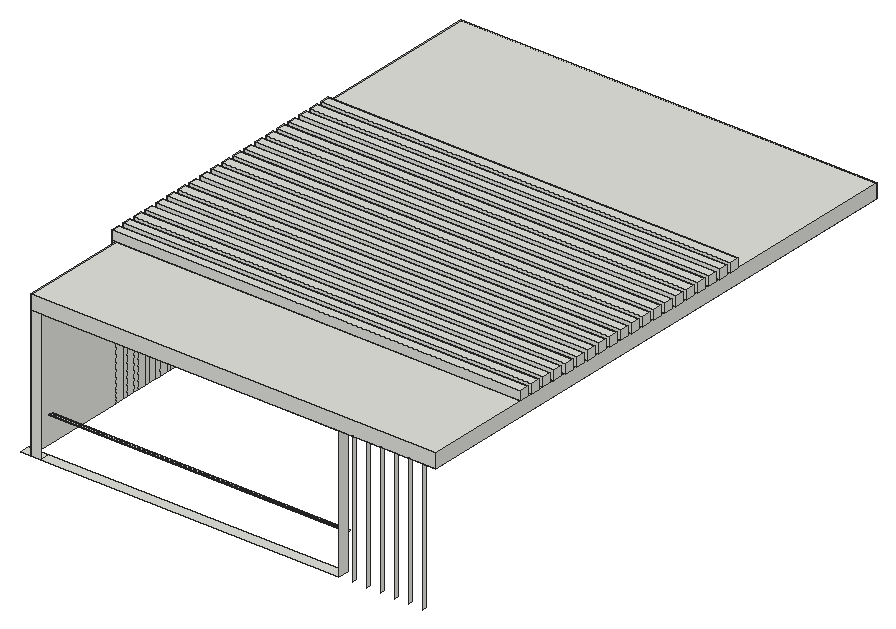
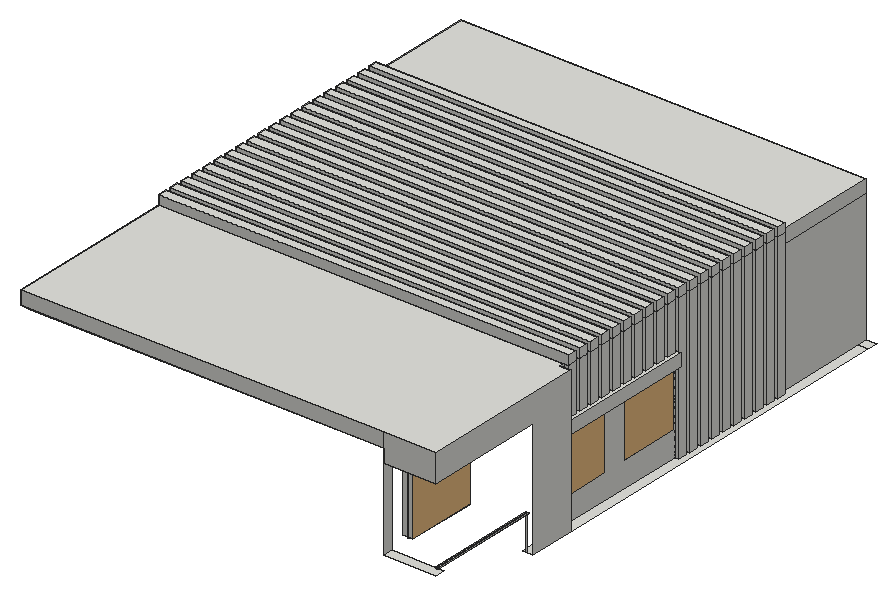
# SketchUp Ruby script. Lengths in inches.
U = 1.inch
M = Sketchup.active_model
def pt(a) = Geom::Point3d.new(a.map { |v| v * U })
def face(e, loops, mat)
  f = e.add_face(loops[0].map { |a| pt(a) })
  loops[1..].each { |l| e.add_face(l.map { |a| pt(a) }).erase! }
  f.material = f.back_material = mat if mat
  f
end
# faces: each face lists its corners as indices into pts; further lists are holes
def faces(e, pts, list, mat = nil) = list.each { |f| face(e, (f[0].is_a?(Array) ? f : [f]).map { |l| l.map { |i| pts[i] } }, mat) }
# xy, xz, yz: faces in a plane at the given z, y or x. An outline is a flat list of corners, or four numbers for a rectangle; further outlines are holes
def ring(l) = l.size == 4 ? [[l[0], l[1]], [l[2], l[1]], [l[2], l[3]], [l[0], l[3]]] : l.each_slice(2).to_a
def flat(e, list, mat, &to3) = list.each { |f| face(e, (f[0].is_a?(Array) ? f : [f]).map { |l| ring(l).map { |u, v| to3.(u, v) } }, mat) }
def xy(e, z, list, mat = nil) = flat(e, list, mat) { |x, y| [x, y, z] }
def xz(e, y, list, mat = nil) = flat(e, list, mat) { |x, z| [x, y, z] }
def yz(e, x, list, mat = nil) = flat(e, list, mat) { |y, z| [x, y, z] }
def lines(e, pts, list) = list.each { |a, b| e.add_line(pt(pts[a]), pt(pts[b])) }
# prism: a flat outline (further loops are holes) pulled along v
def prism(e, loops, v, mat = nil)
  f = face(e, loops, mat); d = Geom::Vector3d.new(v.map { |x| x * U })
  f.pushpull(f.normal.samedirection?(d) ? d.length : -d.length)
end
def box(e, o, s, mat = nil) = prism(e, [[o, [o[0] + s[0], o[1], o[2]], [o[0] + s[0], o[1] + s[1], o[2]], [o[0], o[1] + s[1], o[2]]]], [0, 0, s[2]], mat)
def at(x, y, z, deg = 0) = Geom::Transformation.translation(pt([x, y, z])) * Geom::Transformation.rotation(ORIGIN, Z_AXIS, deg.degrees)
def axes(o, x, y, z) = Geom::Transformation.new([*x, 0, *y, 0, *z, 0, *pt(o).to_a, 1])
def part(name) = M.definitions.add(name)
# library, detail: a bought-in or finely detailed component or shape, given as its bounding box
def library(name, o, s) = part(name).tap { |d| box(d.entities, o, s) }
def detail(e, o, s) = box(e.add_group.entities, o, s)
def put(e, d, t, mat = nil) = e.add_instance(d, t).tap { |i| i.material = mat if mat }
def group(e, t, mat = nil) = e.add_group.tap { |g| g.transformation = t; g.material = mat if mat }.entities
root = M.entities
c1 = library("Window 46-10",[-43.56,-2.12,0],[87.13,4.27,82.67])
xy(root,516,[[16.4375,10.375,25.4375,19.375],[25.4375,10.375,34.4375,19.375],[34.4375,10.375,294.24,19.375],[16.4375,19.375,25.4375,19.375,25.4375,103.4,21.6875,103.4,21.6875,111.11,25.4375,111.11,25.4375,115.4,21.6875,115.4,21.6875,123.11,25.4375,123.11,25.4375,127.4,21.6875,127.4,21.6875,135.11,25.4375,135.11,25.4375,139.4,21.6875,139.4,21.6875,147.11,25.4375,147.11,25.4375,151.4,21.6875,151.4,21.6875,159.11,25.4375,159.11,25.4375,163.4,21.6875,163.4,21.6875,171.11,25.4375,171.11,25.4375,175.4,21.6875,175.4,21.6875,183.11,25.4375,183.11,25.4375,187.4,21.6875,187.4,21.6875,195.11,25.4375,195.11,25.4375,199.4,21.6875,199.4,21.6875,207.11,25.4375,207.11,25.4375,211.4,21.6875,211.4,21.6875,219.11,25.4375,219.11,25.4375,343.55,16.4375,343.55],[21.6875,103.4,25.4375,111.11],
  [21.6875,115.4,25.4375,123.11],[21.6875,127.4,25.4375,135.11],[21.6875,139.4,25.4375,147.11],[21.6875,151.4,25.4375,159.11],[21.6875,163.4,25.4375,171.11],
  [21.6875,175.4,25.4375,183.11],[21.6875,187.4,25.4375,195.11],[21.6875,199.4,25.4375,207.11],[21.6875,211.4,25.4375,219.11],[16.4375,343.55,25.4375,370.6],
  [16.4375,370.6,25.4375,384.4375]])
xy(root,538.43,[[25.4375,221.19,34.4375,272.76],[25.4375,297.07,34.4375,339.01]])
xy(root,544.6,[[61.6875,396.46,70.6875,458.58]])
xy(root,546,[[34.0625,20.75,34.4375,21.125],[34.4375,20.75,34.4375,22.875,34.0625,22.875,34.0625,23.25,292.87,23.25,292.87,20.75],[32.375,21.125,34.0625,22.875],[34.0625,21.125,34.4375,22.875],[20.82,383.57,23.49,481.375],
  [16.4375,481.375,20.82,481.375,20.82,481.49,23.49,481.49,23.49,481.375,61.84,481.375,61.84,490.375,16.4375,490.375],[20.82,481.375,23.49,481.49]])
xy(root,546.5625,[[34.0625,20.75,292.87,23.25]])
xy(root,546.75,[[20.82,383.57,23.49,481.49]])
xy(root,584.75,[[25.4375,221.19,34.4375,272.76],[25.4375,297.07,34.4375,339.01]])
xy(root,589.8,[[18.5,220.25,25.4375,342.75]])
xy(root,598.04,[[61.6875,396.46,70.6875,458.58]])
xy(root,600.93,[[18.5,220.25,25.4375,220.25,25.4375,223.28,21.6875,223.28,21.6875,231.19,25.4375,231.19,25.4375,235.28,21.6875,235.28,21.6875,243.19,25.4375,243.19,25.4375,247.28,21.6875,247.28,21.6875,255.19,25.4375,255.19,25.4375,259.28,21.6875,259.28,21.6875,267.19,25.4375,267.19,25.4375,271.28,21.6875,271.28,21.6875,279.19,25.4375,279.19,25.4375,283.28,21.6875,283.28,21.6875,291.19,25.4375,291.19,25.4375,295.28,21.6875,295.28,21.6875,303.19,25.4375,303.19,25.4375,307.28,21.6875,307.28,21.6875,315.19,25.4375,315.19,25.4375,319.28,21.6875,319.28,21.6875,327.19,25.4375,327.19,25.4375,331.28,21.6875,331.28,21.6875,339.19,25.4375,339.19,25.4375,342.75,18.5,342.75],[21.6875,223.28,25.4375,231.19],[21.6875,235.28,25.4375,243.19],[21.6875,247.28,25.4375,255.19],[21.6875,259.28,25.4375,267.19],
  [21.6875,271.28,25.4375,279.19],[21.6875,283.28,25.4375,291.19],[21.6875,295.28,25.4375,303.19],[21.6875,307.28,25.4375,315.19],[21.6875,319.28,25.4375,327.19],
  [21.6875,331.28,25.4375,339.19]])
xy(root,618.0625,[[16.4375,384.4375,16.4375,490.375,61.84,490.375,61.84,481.375,26.0625,481.375,26.0625,384.4375],[30.13,384.4375,61.6875,477.3]])
xy(root,619.6875,[[26.0625,384.4375,26.0625,481.375,61.6875,481.375,61.6875,477.3,30.13,477.3,30.13,384.4375]])
xy(root,621.1875,[[34.4375,100.375,306.375,109.375]])
xy(root,630,[[25.4375,10.375,34.4375,100.375],[34.4375,10.375,61.84,100.375],[61.84,10.375,61.84,100.375,369.25,100.375,369.25,19.375,294.24,19.375,294.24,10.375],[294.24,10.375,300.62,10.375,300.62,13.75,306.37,13.75,306.37,10.375,312.75,10.375,312.75,13.75,318.49,13.75,318.49,10.375,324.87,10.375,324.87,13.75,330.62,13.75,330.62,10.375,337,10.375,337,13.75,342.74,13.75,342.74,10.375,349.12,10.375,349.12,13.75,354.87,13.75,354.87,10.375,361.25,10.375,361.25,13.75,366.99,13.75,366.99,10.375,369.25,10.375,369.25,19.375,294.24,19.375],[300.62,10.375,306.37,13.75],
  [312.75,10.375,318.49,13.75],[324.87,10.375,330.62,13.75],[337,10.375,342.74,13.75],[349.12,10.375,354.87,13.75],[361.25,10.375,366.99,13.75],
  [369.25,10.375,378.25,490.375],[34.4375,100.375,61.84,109.375],[61.84,100.375,369.25,109.375],[34.4375,109.375,61.84,370.6],[61.84,109.375,61.84,370.6,70.6875,370.6,70.6875,481.375,369.25,481.375,369.25,109.375],
  [61.84,370.6,70.6875,384.4375],[61.6875,384.4375,61.84,481.375],[61.84,384.4375,70.6875,481.375],[61.84,481.375,369.25,490.375]])
xy(root,642,[[25.4375,10.375,378.25,103.4],[21.6875,103.4,25.4375,111.11],[25.4375,103.4,378.25,111.11],[25.4375,111.11,378.25,115.4],[21.6875,115.4,25.4375,123.11],
  [25.4375,115.4,378.25,123.11],[25.4375,123.11,378.25,127.4],[21.6875,127.4,25.4375,135.11],[25.4375,127.4,378.25,135.11],[25.4375,135.11,378.25,139.4],
  [21.6875,139.4,25.4375,147.11],[25.4375,139.4,378.25,147.11],[25.4375,147.11,378.25,151.4],[21.6875,151.4,25.4375,159.11],[25.4375,151.4,378.25,159.11],
  [378.25,151.4,378.625,159.11],[25.4375,159.11,378.25,163.4],[21.6875,163.4,25.4375,171.11],[25.4375,163.4,378.25,171.11],[378.25,163.4,378.625,171.11],
  [25.4375,171.11,378.25,175.4],[21.6875,175.4,25.4375,183.11],[25.4375,175.4,378.25,183.11],[378.25,175.4,378.625,183.11],[25.4375,183.11,378.25,187.4],
  [21.6875,187.4,25.4375,195.11],[25.4375,187.4,378.25,195.11],[378.25,187.4,378.625,195.11],[25.4375,195.11,378.25,199.4],[21.6875,199.4,25.4375,207.11],
  [25.4375,199.4,378.25,207.11],[378.25,199.4,378.625,207.11],[25.4375,207.11,378.25,211.4],[21.6875,211.4,25.4375,219.11],[25.4375,211.4,378.25,219.11],
  [378.25,211.4,378.625,219.11],[25.4375,219.11,378.25,223.28],[21.6875,223.28,25.4375,231.19],[25.4375,223.28,378.25,231.19],[378.25,223.28,378.625,231.19],
  [25.4375,231.19,378.25,235.28],[21.6875,235.28,25.4375,243.19],[25.4375,235.28,378.25,243.19],[378.25,235.28,378.625,243.19],[25.4375,243.19,378.25,247.28],
  [21.6875,247.28,25.4375,255.19],[25.4375,247.28,378.25,255.19],[378.25,247.28,378.625,255.19],[25.4375,255.19,378.25,259.28],[21.6875,259.28,25.4375,267.19],
  [25.4375,259.28,378.25,267.19],[378.25,259.28,378.625,267.19],[25.4375,267.19,378.25,271.28],[21.6875,271.28,25.4375,279.19],[25.4375,271.28,378.25,279.19],
  [378.25,271.28,378.625,279.19],[25.4375,279.19,378.25,283.28],[21.6875,283.28,25.4375,291.19],[25.4375,283.28,378.25,291.19],[378.25,283.28,378.625,291.19],
  [25.4375,291.19,378.25,295.28],[21.6875,295.28,25.4375,303.19],[25.4375,295.28,378.25,303.19],[378.25,295.28,378.625,303.19],[25.4375,303.19,378.25,307.28],
  [21.6875,307.28,25.4375,315.19],[25.4375,307.28,378.25,315.19],[378.25,307.28,378.625,315.19],[25.4375,315.19,378.25,319.28],[21.6875,319.28,25.4375,327.19],
  [25.4375,319.28,378.25,327.19],[378.25,319.28,378.625,327.19],[25.4375,327.19,378.25,331.28],[21.6875,331.28,25.4375,339.19],[25.4375,331.28,378.25,339.19],
  [378.25,331.28,378.625,339.19],[25.4375,339.19,378.25,339.19,378.25,490.375,16.4375,490.375,16.4375,343.55,25.4375,343.55]])
xy(root,650.0625,[[21.6875,103.4,378.25,111.11],[21.6875,115.4,378.25,123.11],[21.6875,127.4,378.25,135.11],[21.6875,139.4,378.25,147.11],[21.6875,151.4,378.625,159.11],
  [21.6875,163.4,378.625,171.11],[21.6875,175.4,378.625,183.11],[21.6875,187.4,378.625,195.11],[21.6875,199.4,378.625,207.11],[21.6875,211.4,378.625,219.11],
  [21.6875,223.28,378.625,231.19],[21.6875,235.28,378.625,243.19],[21.6875,247.28,378.625,255.19],[21.6875,259.28,378.625,267.19],[21.6875,271.28,378.625,279.19],
  [21.6875,283.28,378.625,291.19],[21.6875,295.28,378.625,303.19],[21.6875,307.28,378.625,315.19],[21.6875,319.28,378.625,327.19],[21.6875,331.28,378.625,339.19]])
xz(root,10.375,[[25.4375,516,34.4375,630],[25.4375,630,378.25,642]])
xz(root,20.75,[[34.0625,546,34.4375,546.5625],[34.4375,546,36.1875,546.5625],[36.1875,546,292.87,546.5625]])
xz(root,20.9375,[[36.1875,546,290.56,546.5625]])
xz(root,23.0625,[[36.1875,546,290.56,546.5625]])
xz(root,23.25,[[34.0625,546,36.1875,546.5625],[36.1875,546,292.87,546.5625]])
xz(root,103.4,[[21.6875,516,25.4375,630],[21.6875,630,25.4375,642],[21.6875,642,378.25,650.0625]])
xz(root,111.11,[[21.6875,516,25.4375,642],[21.6875,642,378.25,650.0625]])
xz(root,115.4,[[21.6875,516,25.4375,642],[21.6875,642,378.25,650.0625]])
xz(root,123.11,[[21.6875,516,25.4375,642],[21.6875,642,378.25,650.0625]])
xz(root,127.4,[[21.6875,516,25.4375,642],[21.6875,642,378.25,650.0625]])
xz(root,135.11,[[21.6875,516,25.4375,642],[21.6875,642,378.25,650.0625]])
xz(root,139.4,[[21.6875,516,25.4375,642],[21.6875,642,378.25,650.0625]])
xz(root,147.11,[[21.6875,516,25.4375,642],[21.6875,642,378.25,650.0625]])
xz(root,151.4,[[21.6875,516,25.4375,642],[21.6875,642,378.625,650.0625]])
xz(root,159.11,[[21.6875,516,25.4375,642],[21.6875,642,378.625,650.0625]])
xz(root,163.4,[[21.6875,516,25.4375,642],[21.6875,642,378.625,650.0625]])
xz(root,171.11,[[21.6875,516,25.4375,642],[21.6875,642,378.625,650.0625]])
xz(root,175.4,[[21.6875,516,25.4375,642],[21.6875,642,378.625,650.0625]])
xz(root,183.11,[[21.6875,516,25.4375,642],[21.6875,642,378.625,650.0625]])
xz(root,187.4,[[21.6875,516,25.4375,642],[21.6875,642,378.625,650.0625]])
xz(root,195.11,[[21.6875,516,25.4375,642],[21.6875,642,378.625,650.0625]])
xz(root,199.4,[[21.6875,516,25.4375,642],[21.6875,642,378.625,650.0625]])
xz(root,207.11,[[21.6875,516,25.4375,642],[21.6875,642,378.625,650.0625]])
xz(root,211.4,[[21.6875,516,25.4375,642],[21.6875,642,378.625,650.0625]])
xz(root,219.11,[[21.6875,516,25.4375,642],[21.6875,642,378.625,650.0625]])
xz(root,220.25,[[18.5,589.8,25.4375,600.93]])
xz(root,221.19,[[25.4375,538.43,34.4375,584.75]])
xz(root,223.28,[[21.6875,600.93,25.4375,642],[21.6875,642,378.625,650.0625]])
xz(root,231.19,[[21.6875,600.93,25.4375,642],[21.6875,642,378.625,650.0625]])
xz(root,235.28,[[21.6875,600.93,25.4375,642],[21.6875,642,378.625,650.0625]])
xz(root,243.19,[[21.6875,600.93,25.4375,642],[21.6875,642,378.625,650.0625]])
xz(root,247.28,[[21.6875,600.93,25.4375,642],[21.6875,642,378.625,650.0625]])
xz(root,255.19,[[21.6875,600.93,25.4375,642],[21.6875,642,378.625,650.0625]])
xz(root,259.28,[[21.6875,600.93,25.4375,642],[21.6875,642,378.625,650.0625]])
xz(root,267.19,[[21.6875,600.93,25.4375,642],[21.6875,642,378.625,650.0625]])
xz(root,271.28,[[21.6875,600.93,25.4375,642],[21.6875,642,378.625,650.0625]])
xz(root,272.76,[[25.4375,538.43,34.4375,584.75]])
xz(root,279.19,[[21.6875,600.93,25.4375,642],[21.6875,642,378.625,650.0625]])
xz(root,283.28,[[21.6875,600.93,25.4375,642],[21.6875,642,378.625,650.0625]])
xz(root,291.19,[[21.6875,600.93,25.4375,642],[21.6875,642,378.625,650.0625]])
xz(root,295.28,[[21.6875,600.93,25.4375,642],[21.6875,642,378.625,650.0625]])
xz(root,297.07,[[25.4375,538.43,34.4375,584.75]])
xz(root,303.19,[[21.6875,600.93,25.4375,642],[21.6875,642,378.625,650.0625]])
xz(root,307.28,[[21.6875,600.93,25.4375,642],[21.6875,642,378.625,650.0625]])
xz(root,315.19,[[21.6875,600.93,25.4375,642],[21.6875,642,378.625,650.0625]])
xz(root,319.28,[[21.6875,600.93,25.4375,642],[21.6875,642,378.625,650.0625]])
xz(root,327.19,[[21.6875,600.93,25.4375,642],[21.6875,642,378.625,650.0625]])
xz(root,331.28,[[21.6875,600.93,25.4375,642],[21.6875,642,378.625,650.0625]])
xz(root,339.01,[[25.4375,538.43,34.4375,584.75]])
xz(root,339.19,[[21.6875,600.93,25.4375,642],[21.6875,642,378.625,650.0625]])
xz(root,342.75,[[18.5,589.8,25.4375,600.93]])
xz(root,343.55,[[16.4375,516,25.4375,539.64],[16.4375,539.64,25.4375,630],[16.4375,630,25.4375,642]])
xz(root,383.57,[[20.82,546,23.49,546.75]])
xz(root,384.4375,[[21.68,516,22.63,546]])
xz(root,396.46,[[61.6875,544.6,70.6875,598.04]])
xz(root,458.58,[[61.6875,544.6,70.6875,598.04]])
xz(root,477.3,[[30.13,618.0625,61.6875,619.6875]])
xz(root,481.375,[[61.6875,546,61.84,618.0625],[26.0625,618.0625,61.6875,619.6875],[61.6875,618.0625,61.84,630]])
xz(root,481.49,[[20.82,546,23.49,546.75]])
xz(root,490.375,[[16.4375,618.0625,61.84,642],[61.84,630,378.25,642]])
yz(root,16.4375,[[343.55,516,343.55,642,490.375,642,490.375,618.0625,384.4375,618.0625,384.4375,516]])
yz(root,18.5,[[220.25,589.8,342.75,600.93]])
yz(root,20.82,[[383.57,546,384.4375,546.75],[384.4375,546,481.49,546.75]])
yz(root,21.24,[[385.82,546,479.24,546.75]])
yz(root,21.6875,[[103.4,516,111.11,642],[115.4,516,123.11,642],[127.4,516,135.11,642],[139.4,516,147.11,642],[151.4,516,159.11,642],
  [163.4,516,171.11,642],[175.4,516,183.11,642],[187.4,516,195.11,642],[199.4,516,207.11,642],[211.4,516,219.11,642],
  [223.28,600.93,231.19,642],[235.28,600.93,243.19,642],[247.28,600.93,255.19,642],[259.28,600.93,267.19,642],[271.28,600.93,279.19,642],
  [283.28,600.93,291.19,642],[295.28,600.93,303.19,642],[307.28,600.93,315.19,642],[319.28,600.93,327.19,642],[331.28,600.93,339.19,642],
  [103.4,642,111.11,650.0625],[115.4,642,123.11,650.0625],[127.4,642,135.11,650.0625],[139.4,642,147.11,650.0625],[151.4,642,159.11,650.0625],
  [163.4,642,171.11,650.0625],[175.4,642,183.11,650.0625],[187.4,642,195.11,650.0625],[199.4,642,207.11,650.0625],[211.4,642,219.11,650.0625],
  [223.28,642,231.19,650.0625],[235.28,642,243.19,650.0625],[247.28,642,255.19,650.0625],[259.28,642,267.19,650.0625],[271.28,642,279.19,650.0625],
  [283.28,642,291.19,650.0625],[295.28,642,303.19,650.0625],[307.28,642,315.19,650.0625],[319.28,642,327.19,650.0625],[331.28,642,339.19,650.0625]])
yz(root,23.07,[[385.82,546,479.24,546.75]])
yz(root,23.49,[[383.57,546,481.49,546.75]])
yz(root,25.4375,[[10.375,516,103.4,630],[103.4,516,111.11,642],[111.11,516,115.4,642],[115.4,516,123.11,642],[123.11,516,127.4,642],
  [127.4,516,135.11,642],[135.11,516,139.4,642],[139.4,516,147.11,642],[147.11,516,151.4,642],[151.4,516,159.11,642],
  [159.11,516,163.4,642],[163.4,516,171.11,642],[171.11,516,175.4,642],[175.4,516,183.11,642],[183.11,516,187.4,642],
  [187.4,516,195.11,642],[195.11,516,199.4,642],[199.4,516,207.11,642],[207.11,516,211.4,642],[211.4,516,219.11,642],
  [[219.11,516,219.11,642,223.28,642,223.28,600.93,220.25,600.93,220.25,589.8,342.75,589.8,342.75,600.93,339.19,600.93,339.19,642,343.55,642,343.55,516],[221.19,538.43,272.76,584.75],[297.07,538.43,339.01,584.75]],[220.25,589.8,342.75,600.93],[223.28,600.93,231.19,642],[231.19,600.93,235.28,642],[235.28,600.93,243.19,642],
  [243.19,600.93,247.28,642],[247.28,600.93,255.19,642],[255.19,600.93,259.28,642],[259.28,600.93,267.19,642],[267.19,600.93,271.28,642],
  [271.28,600.93,279.19,642],[279.19,600.93,283.28,642],[283.28,600.93,291.19,642],[291.19,600.93,295.28,642],[295.28,600.93,303.19,642],
  [303.19,600.93,307.28,642],[307.28,600.93,315.19,642],[315.19,600.93,319.28,642],[319.28,600.93,327.19,642],[327.19,600.93,331.28,642],
  [331.28,600.93,339.19,642],[10.375,630,103.4,642]])
yz(root,26.0625,[[384.4375,618.0625,481.375,619.6875]])
yz(root,30.13,[[384.4375,618.0625,477.3,619.6875]])
yz(root,34.0625,[[20.75,546,23.25,546.5625]])
yz(root,34.4375,[[100.375,621.1875,109.375,630]])
yz(root,61.6875,[[384.4375,618.0625,384.4375,630,481.375,630,481.375,619.6875,477.3,619.6875,477.3,618.0625]])
yz(root,61.84,[[481.375,546,490.375,618.0625],[481.375,618.0625,490.375,630]])
yz(root,292.87,[[20.75,546,23.25,546.5625]])
yz(root,294.24,[[10.375,516,19.375,630]])
yz(root,306.37,[[10.375,516,13.75,630]])
yz(root,318.49,[[10.375,516,13.75,630]])
yz(root,330.62,[[10.375,516,13.75,630]])
yz(root,342.74,[[10.375,516,13.75,630]])
yz(root,354.87,[[10.375,516,13.75,630]])
yz(root,366.99,[[10.375,516,13.75,630]])
yz(root,378.25,[[10.375,630,490.375,642],[103.4,642,111.11,650.0625],[115.4,642,123.11,650.0625],[127.4,642,135.11,650.0625],[139.4,642,147.11,650.0625]])
yz(root,378.625,[[151.4,642,159.11,650.0625],[163.4,642,171.11,650.0625],[175.4,642,183.11,650.0625],[187.4,642,195.11,650.0625],[199.4,642,207.11,650.0625],
  [211.4,642,219.11,650.0625],[223.28,642,231.19,650.0625],[235.28,642,243.19,650.0625],[247.28,642,255.19,650.0625],[259.28,642,267.19,650.0625],
  [271.28,642,279.19,650.0625],[283.28,642,291.19,650.0625],[295.28,642,303.19,650.0625],[307.28,642,315.19,650.0625],[319.28,642,327.19,650.0625],
  [331.28,642,339.19,650.0625]])
p = [[61.6875,384.4375,630],[25.4375,384.4375,630],[34.4375,370.6,630],[25.4375,370.6,630],[34.4375,109.375,630],[25.4375,109.375,630]]
lines(root,p,[[0,1],[2,3],[4,5]])
put(root,c1,axes([26.31,318.76,538.35],[0,0.498,0],[-1,0,0],[0,0,0.552]))
put(root,c1,axes([27.58,247.33,538.43],[0,0.6,0],[-1,0,0],[0,0,0.5602]))
put(root,c1,axes([63.83,427.33,544.6],[0,0.71712,0],[-1,0,0],[0,0,0.64639]))
